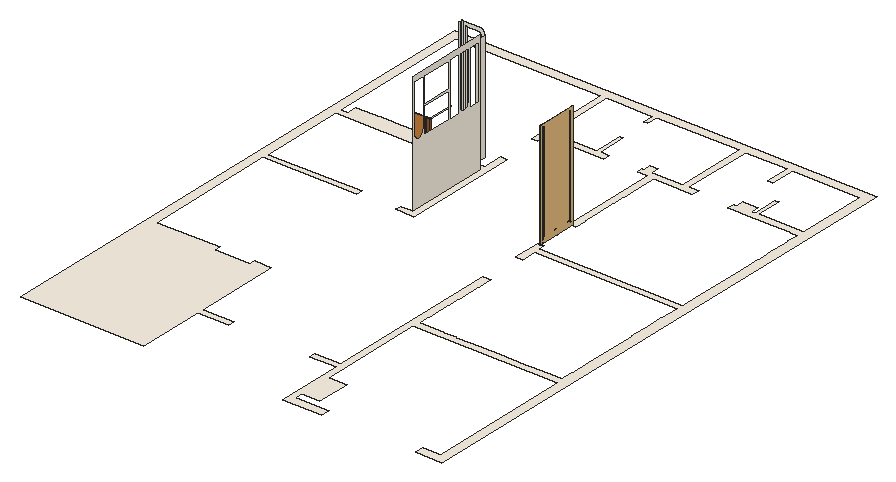
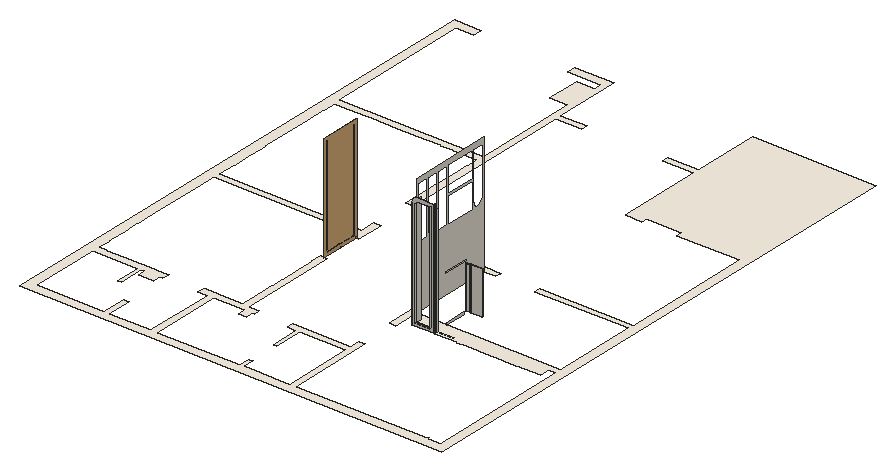
# SketchUp Ruby script. Lengths in inches.
U = 1.inch
M = Sketchup.active_model
def pt(a) = Geom::Point3d.new(a.map { |v| v * U })
def face(e, loops, mat)
  f = e.add_face(loops[0].map { |a| pt(a) })
  loops[1..].each { |l| e.add_face(l.map { |a| pt(a) }).erase! }
  f.material = f.back_material = mat if mat
  f
end
# faces: each face lists its corners as indices into pts; further lists are holes
def faces(e, pts, list, mat = nil) = list.each { |f| face(e, (f[0].is_a?(Array) ? f : [f]).map { |l| l.map { |i| pts[i] } }, mat) }
# xy, xz, yz: faces in a plane at the given z, y or x. An outline is a flat list of corners, or four numbers for a rectangle; further outlines are holes
def ring(l) = l.size == 4 ? [[l[0], l[1]], [l[2], l[1]], [l[2], l[3]], [l[0], l[3]]] : l.each_slice(2).to_a
def flat(e, list, mat, &to3) = list.each { |f| face(e, (f[0].is_a?(Array) ? f : [f]).map { |l| ring(l).map { |u, v| to3.(u, v) } }, mat) }
def xy(e, z, list, mat = nil) = flat(e, list, mat) { |x, y| [x, y, z] }
def xz(e, y, list, mat = nil) = flat(e, list, mat) { |x, z| [x, y, z] }
def yz(e, x, list, mat = nil) = flat(e, list, mat) { |y, z| [x, y, z] }
def lines(e, pts, list) = list.each { |a, b| e.add_line(pt(pts[a]), pt(pts[b])) }
# prism: a flat outline (further loops are holes) pulled along v
def prism(e, loops, v, mat = nil)
  f = face(e, loops, mat); d = Geom::Vector3d.new(v.map { |x| x * U })
  f.pushpull(f.normal.samedirection?(d) ? d.length : -d.length)
end
def box(e, o, s, mat = nil) = prism(e, [[o, [o[0] + s[0], o[1], o[2]], [o[0] + s[0], o[1] + s[1], o[2]], [o[0], o[1] + s[1], o[2]]]], [0, 0, s[2]], mat)
def at(x, y, z, deg = 0) = Geom::Transformation.translation(pt([x, y, z])) * Geom::Transformation.rotation(ORIGIN, Z_AXIS, deg.degrees)
def axes(o, x, y, z) = Geom::Transformation.new([*x, 0, *y, 0, *z, 0, *pt(o).to_a, 1])
def part(name) = M.definitions.add(name)
# library, detail: a bought-in or finely detailed component or shape, given as its bounding box
def library(name, o, s) = part(name).tap { |d| box(d.entities, o, s) }
def detail(e, o, s) = box(e.add_group.entities, o, s)
def put(e, d, t, mat = nil) = e.add_instance(d, t).tap { |i| i.material = mat if mat }
def group(e, t, mat = nil) = e.add_group.tap { |g| g.transformation = t; g.material = mat if mat }.entities
root = M.entities
M.materials.add("Material \#0").color = [86, 53, 35]
M.materials.add("Material \#1").color = [140, 140, 140]
M.materials.add("[0030_OldLace]").color = [253, 245, 230]
M.materials.add("[0040_Peru]").color = [205, 133, 63]
M.materials.add("[Wood Cherry Original]").color = [152, 86, 42]
c1 = part("3DGeom~20_Defintion")
xy(c1.entities,0,[[-976.3,-241.71,-976.3,-223.46,23.7,-241.71],[23.7,-241.71,-976.3,-223.46,5.45,-223.46],[23.7,-241.71,5.45,-223.46,5.45,0],[23.7,-241.71,5.45,0,23.7,0],[-976.3,-223.46,-976.3,-211.85,5.45,-223.46],
  [5.45,-223.46,-976.3,-211.85,-6.16,-211.85],[5.45,-223.46,-6.16,-211.85,-6.16,0],[5.45,-223.46,-6.16,0,5.45,0],[-6.16,0,-6.16,211.85,5.45,223.46],[-6.16,0,5.45,223.46,5.45,0],
  [5.45,0,23.7,241.71,23.7,0],[5.45,0,5.45,223.46,23.7,241.71],[-976.3,211.85,-976.3,223.46,5.45,223.46],[-976.3,211.85,5.45,223.46,-6.16,211.85],[-976.3,223.46,-976.3,241.71,23.7,241.71],
  [-976.3,223.46,23.7,241.71,5.45,223.46]],"Material \#0")
c2 = part("3DGeom~18_Defintion")
xz(c2.entities,-241.71,[[-976.3,0,23.7,0,23.7,7.58],[-976.3,0,23.7,7.58,-976.3,7.58]],"Material \#0")
xz(c2.entities,241.71,[[-976.3,0,-976.3,7.58,23.7,7.58],[-976.3,0,23.7,7.58,23.7,0]],"Material \#0")
yz(c2.entities,23.7,[[-241.71,0,0,0,-241.71,7.58],[0,0,0,7.58,-241.71,7.58],[0,0,241.71,0,241.71,7.58],[0,0,241.71,7.58,0,7.58]],"Material \#0")
c3 = library("3DGeom~16_Defintion",[-962.62,-252.34,-11.22],[1000,504.68,93.46])
c4 = part("3DGeom~22_Defintion")
xz(c4.entities,-210.625,[[-1016.13,2.47,-1016.13,9.96,-16.28,2.47],[-16.28,2.47,-1016.13,9.96,-16.28,9.96],[-1016.13,9.96,-1016.13,51.7,-16.28,51.7],[-1016.13,9.96,-16.28,51.7,-16.28,9.96],[-1016.13,51.7,-1016.13,72.71,-16.28,51.7]],"Material \#0")
xz(c4.entities,210.625,[[-1016.13,2.47,-16.28,2.47,-1016.13,9.96],[-16.28,2.47,-16.28,9.96,-1016.13,9.96],[-1016.13,9.96,-16.28,51.7,-1016.13,51.7],[-1016.13,9.96,-16.28,9.96,-16.28,51.7],[-1016.13,51.7,-16.28,51.7,-1016.13,72.71]],"Material \#0")
yz(c4.entities,-16.28,[[-210.625,2.47,-210.625,9.96,0,9.96],[-210.625,2.47,0,9.96,0,2.47],[0,2.47,0,9.96,210.625,2.47],[210.625,2.47,0,9.96,210.625,9.96],[-210.625,9.96,-210.625,51.7,0,51.7],
  [-210.625,9.96,0,51.7,0,9.96],[0,9.96,0,51.7,210.625,9.96],[210.625,9.96,0,51.7,210.625,51.7],[-210.625,51.7,0,72.71,0,51.7],[0,51.7,0,72.71,210.625,51.7]],"Material \#0")
p = [[-1016.13,-210.625,72.71],[-16.13,-210.77,73.09],[-16.28,-210.625,51.7],[-16.28,-210.625,51.7],[-16.13,-210.77,73.09],[-16.28,0,72.71],
  [-16.13,210.77,73.09],[-16.28,210.625,51.7],[-16.28,210.625,51.7],[-16.13,210.77,73.09],[-1016.13,210.625,72.71]]
faces(c4.entities,p,[[0,1,2],[3,4,5],[5,6,7],[8,9,10]],"Material \#0")
c5 = part("3DGeom~15_Defintion")
xy(c5.entities,0,[[-961.58,-251.9,-958.5,-248.8125,-961.58,-237.8],[-961.58,-251.9,28.8,-248.8125,-958.5,-248.8125],[-961.58,-251.9,36.25,-251.9,28.8,-248.8125],[36.25,-251.9,19.98,-239.99,28.8,-248.8125],[36.25,-251.9,22.16,-237.8,19.98,-239.99],
  [-958.5,-248.8125,-958.5,-237.8,-961.58,-237.8],[19.98,-239.99,22.16,-237.8,3.36,-223.37],[-958.5,-237.8,-958.5,-223.37,-961.58,-220.28],[-961.58,-237.8,-958.5,-237.8,-961.58,-220.28],[22.16,-237.8,4.64,-220.28,3.36,-223.37],
  [-958.5,-223.37,4.64,-220.28,-961.58,-220.28],[-958.5,-223.37,3.36,-223.37,4.64,-220.28],[5.29,-219.63,8.375,-218.35,5.29,0],[8.375,-218.35,8.375,0,5.29,0],[5.29,0,8.375,0,5.29,219.63],
  [8.375,0,8.375,218.35,5.29,219.63],[8.375,218.35,22.8125,237.15,5.29,219.63],[-961.58,220.28,-958.5,223.37,-961.58,237.8],[-961.58,220.28,3.36,223.37,-958.5,223.37],[-961.58,220.28,4.64,220.28,3.36,223.37],
  [4.64,220.28,19.98,239.99,3.36,223.37],[4.64,220.28,22.16,237.8,19.98,239.99],[-958.5,223.37,-958.5,237.8,-961.58,237.8],[-958.5,237.8,-958.5,248.8125,-961.58,251.9],[-961.58,237.8,-958.5,237.8,-961.58,251.9],
  [22.16,237.8,28.8,248.8125,19.98,239.99],[22.16,237.8,36.25,251.9,28.8,248.8125],[-958.5,248.8125,36.25,251.9,-961.58,251.9],[-958.5,248.8125,28.8,248.8125,36.25,251.9]],"Material \#0")
xy(c5.entities,7.48,[[-962.79,-238.36,23.37,-238.36,-962.79,-219.67],[23.37,-238.36,4.67,-219.67,-962.79,-219.67],[23.37,-238.36,23.37,0,4.67,-219.67],[4.67,-219.67,23.37,0,4.67,0],[23.37,0,23.37,238.36,4.67,219.67],
  [4.67,0,23.37,0,4.67,219.67],[-962.79,219.67,23.37,238.36,-962.79,238.36],[-962.79,219.67,4.67,219.67,23.37,238.36]],"Material \#0")
xy(c5.entities,63.5625,[[-962.79,-238.36,-962.79,-219.67,4.67,-219.67],[-962.79,-238.36,4.67,-219.67,23.37,-238.36],[23.37,-238.36,4.67,-219.67,23.37,0],[4.67,-219.67,4.67,0,23.37,0],[23.37,0,4.67,219.67,23.37,238.36],
  [4.67,0,4.67,219.67,23.37,0],[-962.79,219.67,-962.79,238.36,4.67,219.67],[4.67,219.67,-962.79,238.36,23.37,238.36]],"Material \#0")
xy(c5.entities,69.64,[[-962.79,-219.62,4.63,-219.62,-962.79,-200.32],[4.63,-219.62,-14.68,-200.32,-962.79,-200.32],[4.63,-219.62,4.63,0,-14.68,-200.32],[-14.68,-200.32,4.63,0,-14.68,0],[-14.68,0,4.63,0,-14.68,200.32],
  [4.63,0,4.63,219.62,-14.68,200.32],[-962.79,200.32,-14.68,200.32,4.63,219.62],[-962.79,200.32,4.63,219.62,-962.79,219.62]],"Material \#0")
xy(c5.entities,71.04,[[-961.58,-251.9,-958.5,-248.8125,28.8,-248.8125],[-961.58,-251.9,-961.58,-237.8,-958.5,-248.8125],[-961.58,-251.9,28.8,-248.8125,36.25,-251.9],[36.25,-251.9,19.98,-239.99,22.16,-237.8],[36.25,-251.9,28.8,-248.8125,19.98,-239.99],
  [-958.5,-248.8125,-961.58,-237.8,-958.5,-237.8],[19.98,-239.99,3.36,-223.37,22.16,-237.8],[-958.5,-237.8,-961.58,-220.28,-958.5,-223.37],[-961.58,-237.8,-961.58,-220.28,-958.5,-237.8],[22.16,-237.8,3.36,-223.37,4.64,-220.28],
  [-958.5,-223.37,-961.58,-220.28,4.64,-220.28],[-958.5,-223.37,4.64,-220.28,3.36,-223.37],[5.29,-219.63,5.29,0,8.375,-218.35],[8.375,-218.35,5.29,0,8.375,0],[5.29,0,5.29,219.63,8.375,0],
  [8.375,0,5.29,219.63,8.375,218.35],[8.375,218.35,5.29,219.63,22.8125,237.15],[-961.58,220.28,-958.5,223.37,3.36,223.37],[-961.58,220.28,-961.58,237.8,-958.5,223.37],[-961.58,220.28,3.36,223.37,4.64,220.28],
  [4.64,220.28,3.36,223.37,19.98,239.99],[4.64,220.28,19.98,239.99,22.16,237.8],[-958.5,223.37,-961.58,237.8,-958.5,237.8],[-958.5,237.8,-961.58,251.9,-958.5,248.8125],[-961.58,237.8,-961.58,251.9,-958.5,237.8],
  [22.16,237.8,19.98,239.99,28.8,248.8125],[22.16,237.8,28.8,248.8125,36.25,251.9],[-958.5,248.8125,-961.58,251.9,36.25,251.9],[-958.5,248.8125,36.25,251.9,28.8,248.8125]],"Material \#0")
xz(c5.entities,-238.36,[[-962.79,63.5625,23.37,63.5625,23.37,72.07],[-962.79,63.5625,23.37,72.07,-962.79,72.07]],"Material \#0")
xz(c5.entities,-219.67,[[-962.79,7.48,4.67,7.48,-962.79,63.5625],[4.67,7.48,4.67,63.5625,-962.79,63.5625]],"Material \#0")
xz(c5.entities,219.67,[[-962.79,7.48,-962.79,63.5625,4.67,7.48],[4.67,7.48,-962.79,63.5625,4.67,63.5625]],"Material \#0")
xz(c5.entities,238.36,[[-962.79,63.5625,-962.79,72.07,23.37,72.07],[-962.79,63.5625,23.37,72.07,23.37,63.5625]],"Material \#0")
yz(c5.entities,4.67,[[-219.67,7.48,0,7.48,-219.67,63.5625],[0,7.48,0,63.5625,-219.67,63.5625],[0,7.48,219.67,63.5625,0,63.5625],[0,7.48,219.67,7.48,219.67,63.5625]],"Material \#0")
yz(c5.entities,23.37,[[-238.36,63.5625,0,63.5625,-238.36,72.07],[0,63.5625,0,72.07,-238.36,72.07],[0,63.5625,238.36,63.5625,238.36,72.07],[0,63.5625,238.36,72.07,0,72.07]],"Material \#0")
p = [[36.9,-251.24,0],[37.21,0,-0.16],[34.125,0,-0.14],[36.9,251.24,0],[33.83,243.81,0.02],[33.83,-243.8,0.02],
  [22.8125,-237.15,0],[24.99,-234.97,-0.01],[5.375,-220.37,0],[23.37,-238.36,7.48],[4.67,-219.67,7.48],[4.67,-219.67,7.48],
  [23.37,-238.36,7.48],[23.37,-238.36,0],[4.67,-219.67,7.48],[23.37,-238.36,0],[5.375,-220.37,0],[5.375,-220.37,0],
  [23.37,-238.36,0],[5.29,-219.63,0],[8.375,-218.35,0],[-15.36,-199.64,1.62],[4.67,-219.67,7.48],[5.375,-220.37,0],
  [-13.8,-201.19,0.06],[5.375,-220.37,0],[5.375,-220.37,0],[-14.84,-200.15,0.58],[5.375,-220.37,0],[-13.8,-201.19,0.06],
  [-6.08,-208.92,0],[5.375,-220.37,0],[-13.8,-201.19,0.06],[-6.08,-208.92,0],[-13.8,-201.19,0.06],[5.375,-220.37,0],
  [-6.08,-208.92,0],[-13.8,-201.19,0.06],[-13.09,-201.91,0],[-6.08,-208.92,0],[-13.09,-201.91,0],[-13.8,-201.19,0.06],
  [-15.36,199.64,1.62],[4.67,219.67,7.48],[5.375,220.37,0],[-13.8,201.19,0.06],[5.375,220.37,0],[5.375,220.37,0],
  [4.67,219.67,7.48],[-14.84,200.15,0.58],[5.375,220.37,0],[-13.8,201.19,0.06],[-6.08,208.92,0],[-13.09,201.91,0],
  [-13.8,201.19,0.06],[-6.08,208.92,0],[-13.8,201.19,0.06],[5.375,220.37,0],[-6.08,208.92,0],[5.375,220.37,0],
  [-13.8,201.19,0.06],[-6.08,208.92,0],[-13.8,201.19,0.06],[-13.09,201.91,0],[8.375,218.35,0],[24.99,234.97,-0.01],
  [22.8125,237.15,0],[23.37,238.36,7.48],[23.37,238.36,0],[23.37,238.36,0],[5.375,220.37,0],[5.375,220.37,0],
  [23.37,238.36,7.48],[4.67,219.67,7.48],[5.375,220.37,0],[23.37,238.36,0],[23.37,238.36,7.48],[-13.8,-201.19,0.06],
  [-14.84,-200.15,0.58],[-14.38,-200.61,0.26],[-13.8,-201.19,0.06],[-13.8,-201.19,0.06],[-14.38,-200.61,0.26],[-13.8,201.19,0.06],
  [-14.84,200.15,0.58],[-13.8,201.19,0.06],[-14.38,200.61,0.26],[-14.38,200.61,0.26],[-13.8,201.19,0.06],[4.63,-219.62,69.64],
  [4.63,-219.62,69.64],[-15.42,-199.57,9.43],[-15.36,-199.64,1.62],[-15.16,-199.83,1.04],[-15.16,-199.83,1.04],[-15.16,199.83,1.04],
  [-15.36,199.64,1.62],[-15.16,199.83,1.04],[-15.42,199.57,9.43],[4.63,219.62,69.64],[4.67,219.67,7.48],[4.63,219.62,69.64],
  [4.63,-219.62,69.64],[4.67,-219.67,63.5625],[4.67,-219.67,63.5625],[4.67,-219.67,7.48],[-15.28,-199.71,69.25],[4.63,-219.62,69.64],
  [-15.42,-199.57,9.43],[-15.28,-199.71,69.25],[-15.42,-199.57,2.34],[-15.42,-199.57,2.34],[-15.42,199.57,2.34],[-15.42,199.57,9.43],
  [-15.28,199.71,69.25],[-15.28,199.71,69.25],[4.63,219.62,69.64],[4.63,219.62,69.64],[4.67,219.67,63.5625],[4.67,219.67,63.5625],
  [-15.42,199.57,2.34],[4.67,-219.67,63.5625],[4.63,-219.62,69.64],[4.67,219.67,7.48],[4.67,219.67,63.5625],[4.63,219.62,69.64],
  [4.63,-219.62,69.64],[-15.28,-199.71,69.25],[-15.28,-199.71,69.25],[-15.42,-199.57,48.99],[-15.42,-199.57,48.99],[-15.28,-199.71,69.25],
  [-15.42,199.57,48.99],[-15.28,199.71,69.25],[-15.28,199.71,69.25],[-15.42,199.57,48.99],[4.63,219.62,69.64],[4.63,-219.62,69.64],
  [23.37,-238.36,72.07],[4.67,-219.67,63.5625],[4.67,-219.67,63.5625],[23.37,-238.36,63.5625],[23.37,-238.36,72.07],[4.67,-219.67,63.5625],
  [5.24,-220.23,70.03],[23.37,-238.36,72.07],[23.37,-238.36,63.5625],[4.67,-219.67,63.5625],[4.67,-219.67,63.5625],[4.63,-219.62,69.64],
  [4.63,219.62,69.64],[23.37,238.36,72.07],[4.67,219.67,63.5625],[4.67,219.67,63.5625],[5.24,220.23,70.03],[4.63,219.62,69.64],
  [23.37,238.36,63.5625],[4.67,219.67,63.5625],[4.67,219.67,63.5625],[23.37,238.36,63.5625],[23.37,238.36,72.07],[4.67,219.67,63.5625],
  [23.37,238.36,72.07],[4.63,-219.62,69.64],[-14.68,-200.32,69.64],[-15.28,-199.71,69.25],[-15.28,-199.71,69.25],[-14.68,-200.32,69.64],
  [4.63,-219.62,69.64],[-15.28,199.71,69.25],[-14.68,200.32,69.64],[4.63,219.62,69.64],[4.63,219.62,69.64],[-14.68,200.32,69.64],
  [4.63,-219.62,69.64],[5.24,-220.23,70.03],[23.37,-238.36,72.07],[4.63,219.62,69.64],[5.24,220.23,70.03],[5.375,-220.37,72.07],
  [5.375,-220.37,72.07],[23.37,-238.36,72.07],[5.375,220.37,72.07],[23.37,238.36,72.07],[5.375,220.37,72.07],[33.83,-243.8,71.03],
  [36.9,-251.24,71.04],[22.8125,-237.15,71.04],[34.125,0,71.19],[37.21,0,71.2],[24.99,-234.97,71.05],[5.29,-219.63,71.04],
  [8.375,-218.35,71.04],[33.83,243.81,71.03],[36.9,251.24,71.04],[22.8125,237.15,71.04],[24.99,234.97,71.05],[8.375,218.35,71.04]]
faces(c5.entities,p,[[0,1,2],[1,3,4],[4,2,1],[2,5,0],[6,0,5],[5,7,6],[8,9,10],[11,12,13],
  [14,15,16],[17,18,9],[19,6,7],[7,20,19],[21,22,23],[24,21,25],[26,10,27],[28,27,29],
  [30,31,32],[33,34,35],[36,37,38],[39,40,41],[42,43,44],[45,42,46],[47,48,49],[50,49,51],
  [52,53,54],[55,56,57],[58,59,60],[61,62,63],[64,65,66],[43,67,68],[43,69,70],[71,72,73],
  [74,75,76],[3,66,65],[65,4,3],[77,78,21],[27,79,80],[81,82,78],[83,84,42],[85,86,84],
  [49,87,88],[10,89,27],[90,91,27],[92,93,27],[91,92,27],[78,94,21],[84,95,42],[96,97,49],
  [98,96,49],[99,98,49],[100,101,49],[21,102,103],[21,104,105],[21,106,107],[21,108,109],[91,110,92],
  [21,111,108],[42,112,113],[42,113,114],[42,115,116],[42,117,118],[42,119,43],[98,120,96],[10,121,122],
  [123,124,125],[126,127,91],[128,129,91],[108,130,131],[113,132,133],[134,135,98],[136,134,98],[137,138,139],
  [140,141,142],[143,142,144],[145,146,147],[148,144,149],[150,151,152],[153,154,155],[151,156,157],[158,159,160],
  [161,162,154],[163,164,165],[166,167,168],[169,170,171],[172,173,134],[174,175,176],[177,178,151],[142,179,144],
  [175,180,181],[178,182,151],[183,184,154],[185,186,187],[186,185,188],[188,189,186],[187,190,185],[190,187,191],
  [191,192,190],[189,188,193],[193,194,189],[195,196,197],[196,195,194],[194,193,196]],"Material \#0")
c6 = part("3DGeom~19_Defintion")
xy(c6.entities,0,[[-6.28,-215.79,-994.45,-208.55,-13.52,-208.55],[-994.45,-215.79,-994.45,-208.55,-6.28,-215.79],[-6.28,-215.79,-13.52,-208.55,-13.52,0],[-6.28,-215.79,-13.52,0,-6.28,0],[-13.52,0,-13.52,208.55,-6.28,215.79],
  [-13.52,0,-6.28,215.79,-6.28,0],[-994.45,208.55,-6.28,215.79,-13.52,208.55],[-994.45,208.55,-994.45,215.79,-6.28,215.79]],"Material \#0")
p = [[-13.52,-208.55,0],[-994.45,-208.55,0],[-994.45,-207.81,0.07],[-14.25,-207.81,0.07],[-13.52,-208.55,0],[-14.25,-207.81,0.07],
  [-14.25,0,0.07],[-13.52,0,0],[-13.52,208.55,0],[-14.25,207.81,0.07],[-13.52,208.55,0],[-14.25,207.81,0.07],
  [-994.45,207.81,0.07],[-994.45,208.55,0],[-994.45,-207.21,0.27],[-994.45,-207.21,0.27],[-14.86,-207.21,0.27],[-14.86,-207.21,0.27],
  [-14.86,0,0.27],[-14.86,0,0.27],[-14.86,0,0.27],[-14.86,0,0.27],[-14.86,207.21,0.27],[-14.86,207.21,0.27],
  [-994.45,207.21,0.27],[-994.45,207.21,0.27],[-14.86,-207.21,0.27],[-994.45,-207.21,0.27],[-994.45,-206.74,0.6],[-15.33,-206.74,0.6],
  [-14.86,-207.21,0.27],[-15.33,-206.74,0.6],[-15.33,0,0.6],[-14.86,0,0.27],[-14.86,207.21,0.27],[-15.33,206.74,0.6],
  [-14.86,207.21,0.27],[-15.33,206.74,0.6],[-994.45,206.74,0.6],[-994.45,207.21,0.27],[-994.45,-206.4,1.07],[-15.66,-206.4,1.07],
  [-15.66,-206.4,1.07],[-15.66,0,1.07],[-15.66,206.4,1.07],[-15.66,206.4,1.07],[-994.45,206.4,1.07],[-994.45,-206.2,1.68],
  [-15.86,-206.2,1.68],[-15.86,-206.2,1.68],[-15.86,0,1.68],[-15.86,206.2,1.68],[-15.86,206.2,1.68],[-994.45,206.2,1.68],
  [-994.45,-206.13,2.41],[-15.93,-206.13,2.41],[-15.93,-206.13,2.41],[-15.93,0,2.41],[-15.93,206.13,2.41],[-15.93,206.13,2.41],
  [-994.45,206.13,2.41],[-994.45,-206.13,71.16],[-994.45,-206.22,71.59],[-15.79,-206.28,71.53],[-15.79,-206.28,71.53],[-15.84,0,71.59],
  [-15.93,0,71.16],[-15.79,206.28,71.53],[-15.79,206.28,71.53],[-994.45,206.22,71.59],[-994.45,206.13,71.16],[-15.79,-206.28,71.53],
  [-994.45,-206.48,71.84],[-994.45,-206.9,71.93],[-15.16,-206.9,71.93],[-15.79,-206.28,71.53],[-15.79,-206.28,71.53],[-15.16,-206.9,71.93],
  [-15.16,0,71.93],[-994.45,-206.48,71.84],[-15.59,0,71.84],[-15.79,-206.28,71.53],[-15.59,0,71.84],[-15.79,206.28,71.53],
  [-15.16,206.9,71.93],[-15.59,0,71.84],[-15.79,206.28,71.53],[-994.45,206.48,71.84],[-15.79,206.28,71.53],[-15.16,206.9,71.93],
  [-994.45,206.9,71.93],[-994.45,206.48,71.84],[-15.79,206.28,71.53],[-994.45,-227.27,72.01],[5.41,-227.47,72.33],[4.78,-226.84,71.93],
  [4.78,-226.84,71.93],[5.41,-227.47,72.33],[5.21,0,72.01],[-994.45,-226.84,71.93],[-994.45,-227.27,72.01],[5.21,0,72.01],
  [4.78,0,71.93],[4.78,226.84,71.93],[5.21,0,72.01],[5.21,0,72.01],[5.41,227.47,72.33],[4.78,226.84,71.93],
  [5.41,227.47,72.33],[-994.45,227.27,72.01],[-994.45,227.27,72.01],[-994.45,226.84,71.93],[-994.45,-227.27,72.01],[-994.45,-227.53,72.27],
  [5.41,-227.47,72.33],[5.41,-227.47,72.33],[5.47,0,72.27],[5.21,0,72.01],[5.41,227.47,72.33],[5.41,227.47,72.33],
  [-994.45,227.53,72.27],[-994.45,227.27,72.01],[-994.45,-227.61,72.7],[-994.45,-227.61,74.4375],[-994.45,-227.61,74.4375],[5.55,-227.61,74.4375],
  [5.55,-227.61,74.4375],[5.55,0,74.4375],[5.55,0,72.7],[5.55,227.61,74.4375],[5.55,227.61,74.4375],[-994.45,227.61,74.4375],
  [-994.45,227.61,74.4375],[-994.45,227.61,72.7]]
faces(c6.entities,p,[[0,1,2],[2,3,0],[4,5,6],[6,7,4],[8,7,6],[6,9,8],[10,11,12],[12,13,10],
  [3,2,14],[15,16,3],[5,17,18],[19,6,5],[9,6,20],[21,22,9],[11,23,24],[25,12,11],
  [26,27,28],[28,29,26],[30,31,32],[32,33,30],[34,33,32],[32,35,34],[36,37,38],[38,39,36],
  [29,28,40],[40,41,29],[31,42,43],[43,32,31],[35,32,43],[43,44,35],[37,45,46],[46,38,37],
  [41,40,47],[47,48,41],[42,49,50],[50,43,42],[44,43,50],[50,51,44],[45,52,53],[53,46,45],
  [48,47,54],[54,55,48],[49,56,57],[57,50,49],[51,50,57],[57,58,51],[52,59,60],[60,53,52],
  [61,62,63],[64,65,66],[66,65,67],[68,69,70],[71,72,73],[73,74,75],[76,77,78],[62,79,63],
  [78,80,76],[81,82,65],[83,80,78],[78,84,83],[65,85,86],[68,87,69],[88,89,90],[90,91,92],
  [93,94,95],[96,97,98],[95,99,100],[101,102,96],[103,102,104],[105,106,103],[107,108,109],[110,111,107],
  [112,113,114],[115,116,117],[117,116,118],[119,120,121],[114,122,123],[124,125,114],[113,122,114],[115,126,127],
  [127,128,115],[115,128,116],[118,128,127],[127,129,118],[116,128,118],[119,130,131],[132,133,119],[119,133,120]],"Material \#0")
xy(root,0,[[0,4.46,123,4.46,123,71.46,153.875,71.46,153.875,77.46,123,77.46,123,162.9,106.375,162.9,106.375,157.46,9,157.46,9,108.71,9,157.46,71.67,157.46,71.67,162.9,9,162.9,9,295.46,102,295.46,102,301.46,9,301.46,9,385.46,153,385.46,153,301.46,140.9375,301.46,140.9375,295.46,159,295.46,159,411.21,153,411.21,153,391.46,143.9375,391.46,143.9375,402.03,121.95,402.03,121.95,401.46,121.45,401.46,121.45,402.03,99.5625,402.03,99.5625,401.46,99.07,401.46,99.07,402.03,89.9375,402.03,89.9375,401.46,89.38,401.46,89.38,402.03,65.38,402.03,65.38,401.46,64.9,401.46,64.9,402.03,40.64,402.03,40.64,401.46,40.14,401.46,40.14,402.03,16.05,402.03,16.05,391.46,9,391.46,9,535.46,21.4,535.46,21.4,534.59,22.48,534.59,22.48,535.46,153,535.46,153,449.03,159,449.03,159,459.46,217.25,459.46,217.25,465.46,208.56,465.46,208.56,493.9,204.96,493.9,204.96,465.46,159,465.46,159,535.46,204.96,535.46,204.96,524.21,208.56,524.21,208.56,535.46,291,535.46,291,465.46,260.11,465.46,260.11,472.96,252.2,472.96,252.2,465.46,250.125,465.46,250.125,459.46,261,459.46,261,361.78,267.4375,361.78,267.4375,371.96,267,371.96,267,372.47,267.4375,372.47,267.4375,384.44,267,384.44,267,384.9375,267.4375,384.9375,267.4375,408.96,267,408.96,267,409.49,267.4375,409.49,267.4375,421.46,267,421.46,267,421.96,267.4375,421.96,267.4375,445.96,267,445.96,267,446.46,267.4375,446.46,267.4375,458.34,292,458.34,292,459.46,292.51,459.46,292.51,458.34,304.5,458.34,304.5,459.46,305,459.46,305,458.34,306.3125,458.34,306.3125,465.46,297,465.46,297,535.46,339.125,535.46,339.125,511.15,343.94,511.15,343.94,535.46,411,535.46,411,465.46,366.13,465.46,366.13,489.9,362.99,489.9,362.99,465.46,359.6,465.46,359.6,472.4,344.34,472.4,344.34,465.46,341.0625,465.46,341.0625,458.34,341.5,458.34,341.5,459.46,342.01,459.46,342.01,458.34,366,458.34,366,459.46,366.5,459.46,366.5,458.34,378.5,458.34,378.5,459.46,379,459.46,379,458.34,402.99,458.34,402.99,459.46,403.49,459.46,403.49,458.34,410.75,458.34,410.75,446.46,411,446.46,411,445.96,410.75,445.96,410.75,421.96,411,421.96,411,421.46,410.75,421.46,410.75,409.46,411,409.46,411,408.96,410.75,408.96,410.75,384.96,411,384.96,411,384.46,410.75,384.46,410.75,372.46,411,372.46,411,371.96,410.75,371.96,410.75,347.96,411,347.96,411,347.46,410.75,347.46,410.75,335.46,411,335.46,411,334.96,410.75,334.96,410.75,315.46,267.4375,315.46,267.4375,321.88,261,321.88,261,294.63,268.125,294.63,268.125,307.96,267,307.96,267,309.46,410,309.46,410,289.96,411,289.96,411,289.46,410,289.46,410,277.46,411,277.46,411,276.96,410,276.96,410,252.96,411,252.96,411,252.47,410,252.47,410,240.47,411,240.47,411,239.97,410,239.97,410,215.96,411,215.96,411,215.46,410,215.46,410,203.46,411,203.46,411,202.96,410,202.96,410,179,411,179,411,178.44,410,178.44,410,166.15,403,166.15,403,165.46,402.49,165.46,402.49,166.15,378.5,166.15,378.5,165.46,378.01,165.46,378.01,166.15,366,166.15,366,165.46,365.49,165.46,365.49,166.15,341.45,166.15,341.45,165.46,341,165.46,341,166.15,329,166.15,329,165.46,328.5,165.46,328.5,166.15,304.5,166.15,304.5,165.46,304,165.46,304,166.15,292.01,166.15,292.01,165.46,291.48,165.46,291.48,166.15,267.8125,166.15,267.8125,178.47,267,178.47,267,178.96,268.125,178.96,268.125,202.96,267,202.96,267,203.46,268.125,203.46,268.125,215.46,267,215.46,267,215.96,268.125,215.96,268.125,239.96,267,239.96,267,240.46,268.125,240.46,268.125,252.53,267,252.53,267,253,268.125,253,268.125,254.14,261,254.14,261,77.46,234.43,77.46,234.43,71.46,261,71.46,261,4.46,300.25,4.46,300.25,13.46,267,13.46,267,20.99,284.9375,20.99,284.9375,54.35,267,54.35,267,159.46,411,159.46,411,13.46,393.62,13.46,393.62,4.46,420,4.46,420,544.46,0,544.46]],"[0030_OldLace]")
xy(root,2.4375,[[118.29,361.06,118.28,361.93,122.09,361.96,122.1,361.09],[105.79,361.18,105.78,361.93,117.78,361.96,117.79,361.21]],"[0030_OldLace]")
xy(root,2.87,[[102.43,402.03,118.59,402.71]],"[0030_OldLace]")
xy(root,3.39,[[125.33,402.03,140.55,402.71]],"[0030_OldLace]")
xy(root,45.1875,[[105.79,361.18,117.79,361.21,117.78,361.96,105.78,361.93]],"[0040_Peru]")
xy(root,45.1875,[[118.29,361.06,122.1,361.09,122.09,361.96,118.28,361.93]],"[Wood Cherry Original]")
xz(root,401.46,[[121.45,0,121.95,115]],"[0030_OldLace]")
xz(root,402.03,[[[121.95,0,121.95,115,137.86,115,138.66,114.95,139.44,114.79,140.1875,114.54,140.9,114.1875,141.5625,113.74,142.16,113.22,142.68,112.625,143.125,111.96,143.48,111.25,143.73,110.5,143.89,109.72,143.9375,108.93,143.9375,0],[125.33,3.39,140.55,3.39,140.55,108.93,140.53,109.28,140.46,109.62,140.35,109.95,140.19,110.27,140,110.5625,139.76,110.83,139.5,111.06,139.21,111.25,138.89,111.41,138.56,111.52,138.21,111.59,137.86,111.61,125.33,111.61]]],"[0030_OldLace]")
yz(root,118.59,[[402.03,2.87,402.71,112.13]],"[0030_OldLace]")
yz(root,121.45,[[401.46,0,402.03,115]],"[0030_OldLace]")
yz(root,121.95,[[401.46,0,402.03,115]],"[0030_OldLace]")
yz(root,122.59,[[364.03,0,385.46,1.9375]],"[0030_OldLace]")
yz(root,123.52,[[360.6875,45.6875,385.46,46.625]],"[0030_OldLace]")
yz(root,125.33,[[402.03,3.39,402.71,111.61]],"[0030_OldLace]")
yz(root,140.55,[[402.03,3.39,402.71,108.93]],"[0030_OldLace]")
yz(root,143.9375,[[391.46,0,402.03,108.93]],"[0030_OldLace]")
yz(root,153,[[[301.46,0,385.46,120],[315.46,61.54,346.46,87.42],[315.46,88.83,346.46,114.625],[346.96,61.54,358.96,114.625],[371.96,61.54,383.96,114.625],[308.96,61.54,310.36,61.76,311.69,62.4375,312.87,63.52,313.84,64.96,314.55,66.66,314.96,68.56,314.96,114.625,302.96,114.625,302.96,68.56,303.38,66.66,304.09,64.96,305.06,63.52,306.24,62.4375,307.56,61.76],[365.46,61.54,366.86,61.76,368.19,62.4375,369.37,63.52,370.34,64.96,371.05,66.66,371.46,68.56,371.46,114.625,359.46,114.625,359.46,68.56,359.88,66.66,360.59,64.96,361.56,63.52,362.74,62.4375,364.06,61.76]]],"[0030_OldLace]")
yz(root,263.95,[[328.18,50.59,328.18,50.6,328.3,50.6],[328.18,50.6,328.29,50.61,328.3,50.6],[328.22,50.82,328.18,50.83,328.21,50.84],[328.22,50.82,328.21,50.84,328.25,50.84],[328.21,50.84,328.25,50.85,328.25,50.84],
  [328.25,50.84,328.25,50.85,328.29,50.86],[328.25,50.85,328.28,50.87,328.29,50.86],[328.29,50.86,328.28,50.87,328.32,50.89],[328.28,50.87,328.31,50.9,328.32,50.89],[328.32,50.89,328.31,50.9,328.34,50.92],
  [328.31,50.9,328.34,50.93,328.34,50.92],[328.34,50.92,328.34,50.93,328.37,50.96],[328.36,51.24,328.34,51.28,328.34,51.29],[328.36,51.24,328.34,51.29,328.37,51.25],[328.34,51.28,328.31,51.3125,328.32,51.33],
  [328.34,51.28,328.32,51.33,328.34,51.29],[328.31,51.3125,328.28,51.34,328.29,51.35],[328.31,51.3125,328.29,51.35,328.32,51.33],[328.28,51.34,328.25,51.36,328.25,51.375],[328.28,51.34,328.25,51.375,328.29,51.35],
  [328.25,51.36,328.21,51.375,328.22,51.39],[328.25,51.36,328.22,51.39,328.25,51.375],[328.21,51.375,328.18,51.39,328.22,51.39],[328.82,51.46,328.82,53.59,328.83,61.35],[328.82,51.46,328.83,61.35,328.83,51.46],
  [328.82,53.59,328.82,61.35,328.83,61.35]],"Material \#1")
p = [[118.29,361.06,45.1875],[118.29,361.06,2.4375],[122.1,361.09,2.4375],[122.1,361.09,45.1875],[118.28,361.93,45.1875],[118.28,361.93,2.4375],
  [122.09,361.96,2.4375],[122.09,361.96,45.1875],[105.79,361.18,45.1875],[105.79,361.18,2.4375],[117.79,361.21,2.4375],[117.79,361.21,45.1875],
  [105.78,361.93,45.1875],[105.78,361.93,2.4375],[117.78,361.96,2.4375],[117.78,361.96,45.1875]]
faces(root,p,[[0,1,2,3],[4,5,1,0],[6,7,3,2]],"[Wood Cherry Original]")
faces(root,p,[[8,9,10,11],[12,13,9,8],[14,15,11,10]],"[0040_Peru]")
faces(root,p,[[13,12,15,14],[5,4,7,6]],"[0030_OldLace]")
put(root,c1,axes([263.65,342.05,3.9],[0,0,-0.10451],[0,0.07911,0],[0.0054,0,0]),"Material \#0")
put(root,c2,axes([263.65,342.05,3.9],[0,0,-0.10451],[0,0.07911,0],[0.0054,0,0]),"Material \#0")
put(root,c3,axes([263.65,342.05,3.9],[0,0,-0.106],[0,0.08023,0],[0.00548,0,0]),"Material \#0")
put(root,c4,axes([263.65,342.05,3.9],[0,0,-0.10042],[0,0.07601,0],[0.00519,0,0]),"Material \#0")
put(root,c5,axes([263.65,342.05,3.9],[0,0,-0.10598],[0,0.08022,0],[0.00548,0,0]),"Material \#0")
put(root,c6,axes([263.65,342.05,3.9],[0,0,-0.10261],[0,0.07766,0],[0.0053,0,0]),"Material \#0")
